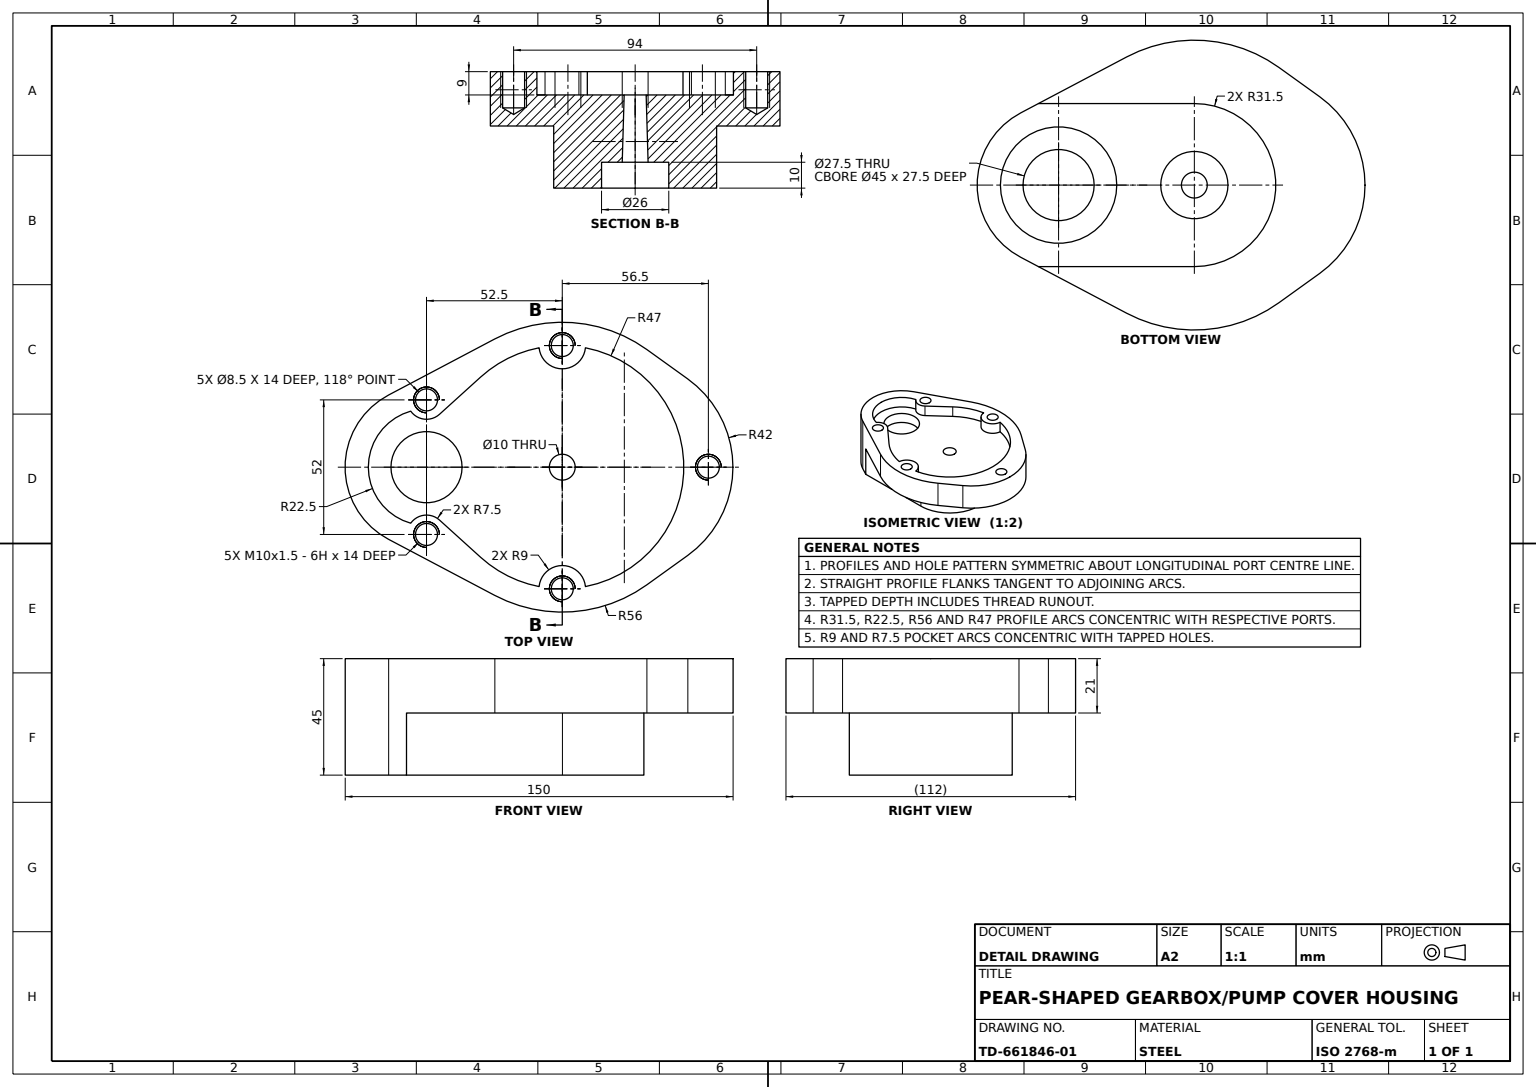
ISO-10303-21;
HEADER;
FILE_DESCRIPTION((''),'2;1');
FILE_NAME('','',(''),(''),'','','');
FILE_SCHEMA(('AUTOMOTIVE_DESIGN'));
ENDSEC;
DATA;
#1=APPLICATION_CONTEXT('');
#2=PRODUCT_CONTEXT('',#1,'mechanical');
#3=PRODUCT('','','',(#2));
#4=PRODUCT_DEFINITION_FORMATION('','',#3);
#5=PRODUCT_DEFINITION_CONTEXT('',#1,'design');
#6=PRODUCT_DEFINITION('','',#4,#5);
#7=PRODUCT_DEFINITION_SHAPE('','',#6);
#8=(LENGTH_UNIT()NAMED_UNIT(*)SI_UNIT(.MILLI.,.METRE.));
#9=(NAMED_UNIT(*)PLANE_ANGLE_UNIT()SI_UNIT($,.RADIAN.));
#10=(NAMED_UNIT(*)SI_UNIT($,.STERADIAN.)SOLID_ANGLE_UNIT());
#11=UNCERTAINTY_MEASURE_WITH_UNIT(LENGTH_MEASURE(1.E-05),#8,'distance_accuracy_value','');
#12=(GEOMETRIC_REPRESENTATION_CONTEXT(3)GLOBAL_UNCERTAINTY_ASSIGNED_CONTEXT((#11))GLOBAL_UNIT_ASSIGNED_CONTEXT((#8,#9,#10))REPRESENTATION_CONTEXT('',''));
#13=CARTESIAN_POINT('',(-26.,4.446342,0.));
#14=VERTEX_POINT('',#13);
#15=CARTESIAN_POINT('',(-26.,7.,4.25));
#16=VERTEX_POINT('',#15);
#17=DIRECTION('',(0.,0.515038075,0.857167301));
#18=VECTOR('',#17,1000.);
#19=LINE('',#15,#18);
#20=EDGE_CURVE('',#14,#16,#19,.T.);
#21=ORIENTED_EDGE('',*,*,#20,.T.);
#22=CARTESIAN_POINT('',(-26.,7.,-4.25));
#23=VERTEX_POINT('',#22);
#24=CARTESIAN_POINT('',(-26.,7.,0.));
#25=DIRECTION('',(0.,1.,0.));
#26=DIRECTION('',(0.,0.,1.));
#27=AXIS2_PLACEMENT_3D('',#24,#25,#26);
#28=CIRCLE('',#27,4.25);
#29=EDGE_CURVE('',#16,#23,#28,.T.);
#30=ORIENTED_EDGE('',*,*,#29,.T.);
#31=DIRECTION('',(0.,0.515038075,-0.857167301));
#32=VECTOR('',#31,1000.);
#33=LINE('',#22,#32);
#34=EDGE_CURVE('',#14,#23,#33,.T.);
#35=ORIENTED_EDGE('',*,*,#34,.F.);
#36=EDGE_LOOP('',(#21,#30,#35));
#37=FACE_OUTER_BOUND('',#36,.T.);
#38=CONICAL_SURFACE('',#27,4.25,1.029744259);
#39=ADVANCED_FACE('',(#37),#38,.F.);
#40=CARTESIAN_POINT('',(0.,21.,-104.75));
#41=VERTEX_POINT('',#40);
#42=CARTESIAN_POINT('',(0.,21.,-113.25));
#43=VERTEX_POINT('',#42);
#44=CARTESIAN_POINT('',(0.,21.,-109.));
#45=AXIS2_PLACEMENT_3D('',#44,#25,#26);
#46=CIRCLE('',#45,4.25);
#47=EDGE_CURVE('',#41,#43,#46,.T.);
#48=ORIENTED_EDGE('',*,*,#47,.T.);
#49=CARTESIAN_POINT('',(0.,7.,-113.25));
#50=VERTEX_POINT('',#49);
#51=VECTOR('',#25,1000.);
#52=LINE('',#42,#51);
#53=EDGE_CURVE('',#50,#43,#52,.T.);
#54=ORIENTED_EDGE('',*,*,#53,.F.);
#55=CARTESIAN_POINT('',(0.,7.,-104.75));
#56=VERTEX_POINT('',#55);
#57=CARTESIAN_POINT('',(0.,7.,-109.));
#58=AXIS2_PLACEMENT_3D('',#57,#25,#26);
#59=CIRCLE('',#58,4.25);
#60=EDGE_CURVE('',#56,#50,#59,.T.);
#61=ORIENTED_EDGE('',*,*,#60,.F.);
#62=LINE('',#40,#51);
#63=EDGE_CURVE('',#56,#41,#62,.T.);
#64=ORIENTED_EDGE('',*,*,#63,.T.);
#65=EDGE_LOOP('',(#48,#54,#61,#64));
#66=FACE_OUTER_BOUND('',#65,.T.);
#67=CYLINDRICAL_SURFACE('',#45,4.25);
#68=ADVANCED_FACE('',(#66),#67,.F.);
#69=CARTESIAN_POINT('',(0.,0.,-118.5));
#70=VERTEX_POINT('',#69);
#71=CARTESIAN_POINT('',(-34.11378,0.,-101.));
#72=VERTEX_POINT('',#71);
#73=CARTESIAN_POINT('',(0.,0.,-76.5));
#74=AXIS2_PLACEMENT_3D('',#73,#25,#26);
#75=CIRCLE('',#74,42.);
#76=EDGE_CURVE('',#70,#72,#75,.T.);
#77=ORIENTED_EDGE('',*,*,#76,.T.);
#78=CARTESIAN_POINT('',(-34.11378,21.,-101.));
#79=VERTEX_POINT('',#78);
#80=DIRECTION('',(0.,-1.,0.));
#81=VECTOR('',#80,1000.);
#82=LINE('',#78,#81);
#83=EDGE_CURVE('',#79,#72,#82,.T.);
#84=ORIENTED_EDGE('',*,*,#83,.F.);
#85=CARTESIAN_POINT('',(0.,21.,-118.5));
#86=VERTEX_POINT('',#85);
#87=CARTESIAN_POINT('',(0.,21.,-76.5));
#88=AXIS2_PLACEMENT_3D('',#87,#25,#26);
#89=CIRCLE('',#88,42.);
#90=EDGE_CURVE('',#86,#79,#89,.T.);
#91=ORIENTED_EDGE('',*,*,#90,.F.);
#92=LINE('',#85,#81);
#93=EDGE_CURVE('',#86,#70,#92,.T.);
#94=ORIENTED_EDGE('',*,*,#93,.T.);
#95=EDGE_LOOP('',(#77,#84,#91,#94));
#96=FACE_OUTER_BOUND('',#95,.T.);
#97=DIRECTION('',(0.,0.,-1.));
#98=AXIS2_PLACEMENT_3D('',#87,#80,#97);
#99=CYLINDRICAL_SURFACE('',#98,42.);
#100=ADVANCED_FACE('',(#96),#99,.T.);
#101=CARTESIAN_POINT('',(0.,12.,-47.5));
#102=VERTEX_POINT('',#101);
#103=CARTESIAN_POINT('',(0.,-14.,-47.5));
#104=VERTEX_POINT('',#103);
#105=CARTESIAN_POINT('',(0.,-24.,-47.5));
#106=LINE('',#105,#81);
#107=EDGE_CURVE('',#102,#104,#106,.T.);
#108=ORIENTED_EDGE('',*,*,#107,.T.);
#109=CARTESIAN_POINT('',(0.,-14.,-57.5));
#110=VERTEX_POINT('',#109);
#111=CARTESIAN_POINT('',(0.,-14.,-52.5));
#112=AXIS2_PLACEMENT_3D('',#111,#80,#97);
#113=CIRCLE('',#112,5.);
#114=EDGE_CURVE('',#104,#110,#113,.T.);
#115=ORIENTED_EDGE('',*,*,#114,.T.);
#116=CARTESIAN_POINT('',(0.,12.,-57.5));
#117=VERTEX_POINT('',#116);
#118=CARTESIAN_POINT('',(0.,-24.,-57.5));
#119=LINE('',#118,#81);
#120=EDGE_CURVE('',#117,#110,#119,.T.);
#121=ORIENTED_EDGE('',*,*,#120,.F.);
#122=CARTESIAN_POINT('',(0.,12.,-52.5));
#123=AXIS2_PLACEMENT_3D('',#122,#25,#26);
#124=CIRCLE('',#123,5.);
#125=EDGE_CURVE('',#117,#102,#124,.T.);
#126=ORIENTED_EDGE('',*,*,#125,.T.);
#127=EDGE_LOOP('',(#108,#115,#121,#126));
#128=FACE_OUTER_BOUND('',#127,.T.);
#129=CARTESIAN_POINT('',(0.,-24.,-52.5));
#130=AXIS2_PLACEMENT_3D('',#129,#80,#97);
#131=CYLINDRICAL_SURFACE('',#130,5.);
#132=ADVANCED_FACE('',(#128),#131,.F.);
#133=CARTESIAN_POINT('',(-47.,21.,-48.25));
#134=VERTEX_POINT('',#133);
#135=CARTESIAN_POINT('',(-47.,21.,-56.75));
#136=VERTEX_POINT('',#135);
#137=CARTESIAN_POINT('',(-47.,21.,-52.5));
#138=AXIS2_PLACEMENT_3D('',#137,#25,#26);
#139=CIRCLE('',#138,4.25);
#140=EDGE_CURVE('',#134,#136,#139,.T.);
#141=ORIENTED_EDGE('',*,*,#140,.T.);
#142=CARTESIAN_POINT('',(-47.,7.,-56.75));
#143=VERTEX_POINT('',#142);
#144=LINE('',#135,#51);
#145=EDGE_CURVE('',#143,#136,#144,.T.);
#146=ORIENTED_EDGE('',*,*,#145,.F.);
#147=CARTESIAN_POINT('',(-47.,7.,-48.25));
#148=VERTEX_POINT('',#147);
#149=CARTESIAN_POINT('',(-47.,7.,-52.5));
#150=AXIS2_PLACEMENT_3D('',#149,#25,#26);
#151=CIRCLE('',#150,4.25);
#152=EDGE_CURVE('',#148,#143,#151,.T.);
#153=ORIENTED_EDGE('',*,*,#152,.F.);
#154=LINE('',#133,#51);
#155=EDGE_CURVE('',#148,#134,#154,.T.);
#156=ORIENTED_EDGE('',*,*,#155,.T.);
#157=EDGE_LOOP('',(#141,#146,#153,#156));
#158=FACE_OUTER_BOUND('',#157,.T.);
#159=CYLINDRICAL_SURFACE('',#138,4.25);
#160=ADVANCED_FACE('',(#158),#159,.F.);
#161=CARTESIAN_POINT('',(-26.,21.,-4.25));
#162=VERTEX_POINT('',#161);
#163=LINE('',#161,#51);
#164=EDGE_CURVE('',#23,#162,#163,.T.);
#165=ORIENTED_EDGE('',*,*,#164,.T.);
#166=CARTESIAN_POINT('',(-26.,21.,4.25));
#167=VERTEX_POINT('',#166);
#168=CARTESIAN_POINT('',(-26.,21.,0.));
#169=AXIS2_PLACEMENT_3D('',#168,#25,#26);
#170=CIRCLE('',#169,4.25);
#171=EDGE_CURVE('',#162,#167,#170,.T.);
#172=ORIENTED_EDGE('',*,*,#171,.T.);
#173=LINE('',#166,#51);
#174=EDGE_CURVE('',#16,#167,#173,.T.);
#175=ORIENTED_EDGE('',*,*,#174,.F.);
#176=EDGE_CURVE('',#23,#16,#28,.T.);
#177=ORIENTED_EDGE('',*,*,#176,.F.);
#178=EDGE_LOOP('',(#165,#172,#175,#177));
#179=FACE_OUTER_BOUND('',#178,.T.);
#180=CYLINDRICAL_SURFACE('',#169,4.25);
#181=ADVANCED_FACE('',(#179),#180,.F.);
#182=CARTESIAN_POINT('',(-21.653846,12.,6.11236));
#183=VERTEX_POINT('',#182);
#184=CARTESIAN_POINT('',(0.,12.,22.5));
#185=VERTEX_POINT('',#184);
#186=CARTESIAN_POINT('',(0.,12.,0.));
#187=AXIS2_PLACEMENT_3D('',#186,#25,#26);
#188=CIRCLE('',#187,22.5);
#189=EDGE_CURVE('',#183,#185,#188,.T.);
#190=ORIENTED_EDGE('',*,*,#189,.F.);
#191=CARTESIAN_POINT('',(-21.653846,21.,6.11236));
#192=VERTEX_POINT('',#191);
#193=LINE('',#182,#51);
#194=EDGE_CURVE('',#183,#192,#193,.T.);
#195=ORIENTED_EDGE('',*,*,#194,.T.);
#196=CARTESIAN_POINT('',(0.,21.,22.5));
#197=VERTEX_POINT('',#196);
#198=CARTESIAN_POINT('',(0.,21.,0.));
#199=AXIS2_PLACEMENT_3D('',#198,#25,#26);
#200=CIRCLE('',#199,22.5);
#201=EDGE_CURVE('',#192,#197,#200,.T.);
#202=ORIENTED_EDGE('',*,*,#201,.T.);
#203=LINE('',#184,#51);
#204=EDGE_CURVE('',#185,#197,#203,.T.);
#205=ORIENTED_EDGE('',*,*,#204,.F.);
#206=EDGE_LOOP('',(#190,#195,#202,#205));
#207=FACE_OUTER_BOUND('',#206,.T.);
#208=CYLINDRICAL_SURFACE('',#187,22.5);
#209=ADVANCED_FACE('',(#207),#208,.F.);
#210=CARTESIAN_POINT('',(-49.528264,21.,-26.366667));
#211=VERTEX_POINT('',#210);
#212=CARTESIAN_POINT('',(-49.528264,0.,-26.366667));
#213=VERTEX_POINT('',#212);
#214=LINE('',#210,#81);
#215=EDGE_CURVE('',#211,#213,#214,.T.);
#216=ORIENTED_EDGE('',*,*,#215,.F.);
#217=CARTESIAN_POINT('',(-45.48504,21.,-85.166667));
#218=VERTEX_POINT('',#217);
#219=CARTESIAN_POINT('',(0.,21.,-52.5));
#220=AXIS2_PLACEMENT_3D('',#219,#25,#26);
#221=CIRCLE('',#220,56.);
#222=EDGE_CURVE('',#218,#211,#221,.T.);
#223=ORIENTED_EDGE('',*,*,#222,.F.);
#224=CARTESIAN_POINT('',(-45.48504,0.,-85.166667));
#225=VERTEX_POINT('',#224);
#226=LINE('',#217,#81);
#227=EDGE_CURVE('',#218,#225,#226,.T.);
#228=ORIENTED_EDGE('',*,*,#227,.T.);
#229=CARTESIAN_POINT('',(0.,0.,-52.5));
#230=AXIS2_PLACEMENT_3D('',#229,#25,#26);
#231=CIRCLE('',#230,56.);
#232=EDGE_CURVE('',#225,#213,#231,.T.);
#233=ORIENTED_EDGE('',*,*,#232,.T.);
#234=EDGE_LOOP('',(#216,#223,#228,#233));
#235=FACE_OUTER_BOUND('',#234,.T.);
#236=AXIS2_PLACEMENT_3D('',#219,#80,#97);
#237=CYLINDRICAL_SURFACE('',#236,56.);
#238=ADVANCED_FACE('',(#235),#237,.T.);
#239=ORIENTED_EDGE('',*,*,#204,.T.);
#240=CARTESIAN_POINT('',(21.653846,21.,6.11236));
#241=VERTEX_POINT('',#240);
#242=EDGE_CURVE('',#197,#241,#200,.T.);
#243=ORIENTED_EDGE('',*,*,#242,.T.);
#244=CARTESIAN_POINT('',(21.653846,12.,6.11236));
#245=VERTEX_POINT('',#244);
#246=LINE('',#244,#51);
#247=EDGE_CURVE('',#245,#241,#246,.T.);
#248=ORIENTED_EDGE('',*,*,#247,.F.);
#249=EDGE_CURVE('',#185,#245,#188,.T.);
#250=ORIENTED_EDGE('',*,*,#249,.F.);
#251=EDGE_LOOP('',(#239,#243,#248,#250));
#252=FACE_OUTER_BOUND('',#251,.T.);
#253=ADVANCED_FACE('',(#252),#208,.F.);
#254=CARTESIAN_POINT('',(-46.138298,12.,-43.541347));
#255=VERTEX_POINT('',#254);
#256=CARTESIAN_POINT('',(-46.138298,21.,-43.541347));
#257=VERTEX_POINT('',#256);
#258=LINE('',#254,#51);
#259=EDGE_CURVE('',#255,#257,#258,.T.);
#260=ORIENTED_EDGE('',*,*,#259,.T.);
#261=CARTESIAN_POINT('',(-34.856407,21.,-20.971744));
#262=VERTEX_POINT('',#261);
#263=CIRCLE('',#220,47.);
#264=EDGE_CURVE('',#257,#262,#263,.T.);
#265=ORIENTED_EDGE('',*,*,#264,.T.);
#266=CARTESIAN_POINT('',(-34.856407,12.,-20.971744));
#267=VERTEX_POINT('',#266);
#268=LINE('',#266,#51);
#269=EDGE_CURVE('',#267,#262,#268,.T.);
#270=ORIENTED_EDGE('',*,*,#269,.F.);
#271=CIRCLE('',#123,47.);
#272=EDGE_CURVE('',#255,#267,#271,.T.);
#273=ORIENTED_EDGE('',*,*,#272,.F.);
#274=EDGE_LOOP('',(#260,#265,#270,#273));
#275=FACE_OUTER_BOUND('',#274,.T.);
#276=CYLINDRICAL_SURFACE('',#123,47.);
#277=ADVANCED_FACE('',(#275),#276,.F.);
#278=CARTESIAN_POINT('',(26.,4.446342,0.));
#279=VERTEX_POINT('',#278);
#280=CARTESIAN_POINT('',(26.,7.,4.25));
#281=VERTEX_POINT('',#280);
#282=LINE('',#280,#18);
#283=EDGE_CURVE('',#279,#281,#282,.T.);
#284=ORIENTED_EDGE('',*,*,#283,.T.);
#285=CARTESIAN_POINT('',(26.,7.,-4.25));
#286=VERTEX_POINT('',#285);
#287=CARTESIAN_POINT('',(26.,7.,0.));
#288=AXIS2_PLACEMENT_3D('',#287,#25,#26);
#289=CIRCLE('',#288,4.25);
#290=EDGE_CURVE('',#281,#286,#289,.T.);
#291=ORIENTED_EDGE('',*,*,#290,.T.);
#292=LINE('',#285,#32);
#293=EDGE_CURVE('',#279,#286,#292,.T.);
#294=ORIENTED_EDGE('',*,*,#293,.F.);
#295=EDGE_LOOP('',(#284,#291,#294));
#296=FACE_OUTER_BOUND('',#295,.T.);
#297=CONICAL_SURFACE('',#288,4.25,1.029744259);
#298=ADVANCED_FACE('',(#296),#297,.F.);
#299=CARTESIAN_POINT('',(47.,7.,-56.75));
#300=VERTEX_POINT('',#299);
#301=CARTESIAN_POINT('',(47.,21.,-56.75));
#302=VERTEX_POINT('',#301);
#303=LINE('',#301,#51);
#304=EDGE_CURVE('',#300,#302,#303,.T.);
#305=ORIENTED_EDGE('',*,*,#304,.F.);
#306=CARTESIAN_POINT('',(47.,7.,-48.25));
#307=VERTEX_POINT('',#306);
#308=CARTESIAN_POINT('',(47.,7.,-52.5));
#309=AXIS2_PLACEMENT_3D('',#308,#25,#26);
#310=CIRCLE('',#309,4.25);
#311=EDGE_CURVE('',#307,#300,#310,.T.);
#312=ORIENTED_EDGE('',*,*,#311,.F.);
#313=CARTESIAN_POINT('',(47.,21.,-48.25));
#314=VERTEX_POINT('',#313);
#315=LINE('',#313,#51);
#316=EDGE_CURVE('',#307,#314,#315,.T.);
#317=ORIENTED_EDGE('',*,*,#316,.T.);
#318=CARTESIAN_POINT('',(47.,21.,-52.5));
#319=AXIS2_PLACEMENT_3D('',#318,#25,#26);
#320=CIRCLE('',#319,4.25);
#321=EDGE_CURVE('',#314,#302,#320,.T.);
#322=ORIENTED_EDGE('',*,*,#321,.T.);
#323=EDGE_LOOP('',(#305,#312,#317,#322));
#324=FACE_OUTER_BOUND('',#323,.T.);
#325=CYLINDRICAL_SURFACE('',#319,4.25);
#326=ADVANCED_FACE('',(#324),#325,.F.);
#327=CARTESIAN_POINT('',(0.,-24.,-65.5));
#328=VERTEX_POINT('',#327);
#329=CARTESIAN_POINT('',(0.,-24.,-39.5));
#330=VERTEX_POINT('',#329);
#331=CIRCLE('',#130,13.);
#332=EDGE_CURVE('',#328,#330,#331,.T.);
#333=ORIENTED_EDGE('',*,*,#332,.T.);
#334=CARTESIAN_POINT('',(0.,-14.,-39.5));
#335=VERTEX_POINT('',#334);
#336=LINE('',#329,#81);
#337=EDGE_CURVE('',#335,#330,#336,.T.);
#338=ORIENTED_EDGE('',*,*,#337,.F.);
#339=CARTESIAN_POINT('',(0.,-14.,-65.5));
#340=VERTEX_POINT('',#339);
#341=CIRCLE('',#112,13.);
#342=EDGE_CURVE('',#340,#335,#341,.T.);
#343=ORIENTED_EDGE('',*,*,#342,.F.);
#344=LINE('',#327,#81);
#345=EDGE_CURVE('',#340,#328,#344,.T.);
#346=ORIENTED_EDGE('',*,*,#345,.T.);
#347=EDGE_LOOP('',(#333,#338,#343,#346));
#348=FACE_OUTER_BOUND('',#347,.T.);
#349=CYLINDRICAL_SURFACE('',#130,13.);
#350=ADVANCED_FACE('',(#348),#349,.F.);
#351=CARTESIAN_POINT('',(0.,4.446342,-109.));
#352=VERTEX_POINT('',#351);
#353=LINE('',#55,#18);
#354=EDGE_CURVE('',#352,#56,#353,.T.);
#355=ORIENTED_EDGE('',*,*,#354,.F.);
#356=LINE('',#49,#32);
#357=EDGE_CURVE('',#352,#50,#356,.T.);
#358=ORIENTED_EDGE('',*,*,#357,.T.);
#359=EDGE_CURVE('',#50,#56,#59,.T.);
#360=ORIENTED_EDGE('',*,*,#359,.T.);
#361=EDGE_LOOP('',(#355,#358,#360));
#362=FACE_OUTER_BOUND('',#361,.T.);
#363=CONICAL_SURFACE('',#58,4.25,1.029744259);
#364=ADVANCED_FACE('',(#362),#363,.F.);
#365=CARTESIAN_POINT('',(-46.138298,12.,-61.458653));
#366=VERTEX_POINT('',#365);
#367=CARTESIAN_POINT('',(-47.,12.,-52.5));
#368=AXIS2_PLACEMENT_3D('',#367,#80,#26);
#369=CIRCLE('',#368,9.);
#370=EDGE_CURVE('',#366,#255,#369,.T.);
#371=ORIENTED_EDGE('',*,*,#370,.F.);
#372=CARTESIAN_POINT('',(-46.138298,21.,-61.458653));
#373=VERTEX_POINT('',#372);
#374=LINE('',#365,#51);
#375=EDGE_CURVE('',#366,#373,#374,.T.);
#376=ORIENTED_EDGE('',*,*,#375,.T.);
#377=AXIS2_PLACEMENT_3D('',#137,#80,#26);
#378=CIRCLE('',#377,9.);
#379=EDGE_CURVE('',#373,#257,#378,.T.);
#380=ORIENTED_EDGE('',*,*,#379,.T.);
#381=ORIENTED_EDGE('',*,*,#259,.F.);
#382=EDGE_LOOP('',(#371,#376,#380,#381));
#383=FACE_OUTER_BOUND('',#382,.T.);
#384=AXIS2_PLACEMENT_3D('',#367,#25,#26);
#385=CYLINDRICAL_SURFACE('',#384,9.);
#386=ADVANCED_FACE('',(#383),#385,.T.);
#387=ORIENTED_EDGE('',*,*,#120,.T.);
#388=EDGE_CURVE('',#110,#104,#113,.T.);
#389=ORIENTED_EDGE('',*,*,#388,.T.);
#390=ORIENTED_EDGE('',*,*,#107,.F.);
#391=EDGE_CURVE('',#102,#117,#124,.T.);
#392=ORIENTED_EDGE('',*,*,#391,.T.);
#393=EDGE_LOOP('',(#387,#389,#390,#392));
#394=FACE_OUTER_BOUND('',#393,.T.);
#395=ADVANCED_FACE('',(#394),#131,.F.);
#396=ORIENTED_EDGE('',*,*,#176,.T.);
#397=ORIENTED_EDGE('',*,*,#20,.F.);
#398=ORIENTED_EDGE('',*,*,#34,.T.);
#399=EDGE_LOOP('',(#396,#397,#398));
#400=FACE_OUTER_BOUND('',#399,.T.);
#401=ADVANCED_FACE('',(#400),#38,.F.);
#402=CARTESIAN_POINT('',(-47.,4.446342,-52.5));
#403=VERTEX_POINT('',#402);
#404=LINE('',#142,#32);
#405=EDGE_CURVE('',#403,#143,#404,.T.);
#406=ORIENTED_EDGE('',*,*,#405,.T.);
#407=EDGE_CURVE('',#143,#148,#151,.T.);
#408=ORIENTED_EDGE('',*,*,#407,.T.);
#409=LINE('',#147,#18);
#410=EDGE_CURVE('',#403,#148,#409,.T.);
#411=ORIENTED_EDGE('',*,*,#410,.F.);
#412=EDGE_LOOP('',(#406,#408,#411));
#413=FACE_OUTER_BOUND('',#412,.T.);
#414=CONICAL_SURFACE('',#150,4.25,1.029744259);
#415=ADVANCED_FACE('',(#413),#414,.F.);
#416=ORIENTED_EDGE('',*,*,#227,.F.);
#417=DIRECTION('',(-0.583333333,0.,0.812232862));
#418=VECTOR('',#417,1000.);
#419=LINE('',#217,#418);
#420=EDGE_CURVE('',#79,#218,#419,.T.);
#421=ORIENTED_EDGE('',*,*,#420,.F.);
#422=ORIENTED_EDGE('',*,*,#83,.T.);
#423=LINE('',#224,#418);
#424=EDGE_CURVE('',#72,#225,#423,.T.);
#425=ORIENTED_EDGE('',*,*,#424,.T.);
#426=EDGE_LOOP('',(#416,#421,#422,#425));
#427=FACE_OUTER_BOUND('',#426,.T.);
#428=DIRECTION('',(0.812232862,0.,0.583333333));
#429=DIRECTION('',(0.583333333,0.,-0.812232862));
#430=AXIS2_PLACEMENT_3D('',#217,#428,#429);
#431=PLANE('',#430);
#432=ADVANCED_FACE('',(#427),#431,.F.);
#433=ORIENTED_EDGE('',*,*,#332,.F.);
#434=EDGE_CURVE('',#330,#328,#331,.T.);
#435=ORIENTED_EDGE('',*,*,#434,.F.);
#436=EDGE_LOOP('',(#433,#435));
#437=FACE_BOUND('',#436,.T.);
#438=CARTESIAN_POINT('',(0.,-24.,-22.5));
#439=VERTEX_POINT('',#438);
#440=CARTESIAN_POINT('',(0.,-24.,22.5));
#441=VERTEX_POINT('',#440);
#442=CARTESIAN_POINT('',(0.,-24.,0.));
#443=AXIS2_PLACEMENT_3D('',#442,#80,#97);
#444=CIRCLE('',#443,22.5);
#445=EDGE_CURVE('',#439,#441,#444,.T.);
#446=ORIENTED_EDGE('',*,*,#445,.F.);
#447=EDGE_CURVE('',#441,#439,#444,.T.);
#448=ORIENTED_EDGE('',*,*,#447,.F.);
#449=EDGE_LOOP('',(#446,#448));
#450=FACE_BOUND('',#449,.T.);
#451=CARTESIAN_POINT('',(-27.859648,-24.,14.7));
#452=VERTEX_POINT('',#451);
#453=CARTESIAN_POINT('',(-31.5,-24.,7.800754));
#454=VERTEX_POINT('',#453);
#455=DIRECTION('',(-0.466666667,0.,-0.884433277));
#456=VECTOR('',#455,1000.);
#457=LINE('',#453,#456);
#458=EDGE_CURVE('',#452,#454,#457,.T.);
#459=ORIENTED_EDGE('',*,*,#458,.T.);
#460=CARTESIAN_POINT('',(-31.5,-24.,-52.5));
#461=VERTEX_POINT('',#460);
#462=CARTESIAN_POINT('',(-31.5,-24.,0.));
#463=VECTOR('',#97,1000.);
#464=LINE('',#462,#463);
#465=EDGE_CURVE('',#454,#461,#464,.T.);
#466=ORIENTED_EDGE('',*,*,#465,.T.);
#467=CARTESIAN_POINT('',(31.5,-24.,-52.5));
#468=VERTEX_POINT('',#467);
#469=CIRCLE('',#130,31.5);
#470=EDGE_CURVE('',#461,#468,#469,.T.);
#471=ORIENTED_EDGE('',*,*,#470,.T.);
#472=CARTESIAN_POINT('',(31.5,-24.,7.800754));
#473=VERTEX_POINT('',#472);
#474=CARTESIAN_POINT('',(31.5,-24.,0.));
#475=VECTOR('',#26,1000.);
#476=LINE('',#474,#475);
#477=EDGE_CURVE('',#468,#473,#476,.T.);
#478=ORIENTED_EDGE('',*,*,#477,.T.);
#479=CARTESIAN_POINT('',(27.859648,-24.,14.7));
#480=VERTEX_POINT('',#479);
#481=DIRECTION('',(-0.466666667,0.,0.884433277));
#482=VECTOR('',#481,1000.);
#483=LINE('',#479,#482);
#484=EDGE_CURVE('',#473,#480,#483,.T.);
#485=ORIENTED_EDGE('',*,*,#484,.T.);
#486=CIRCLE('',#443,31.5);
#487=EDGE_CURVE('',#480,#452,#486,.T.);
#488=ORIENTED_EDGE('',*,*,#487,.T.);
#489=EDGE_LOOP('',(#459,#466,#471,#478,#485,#488));
#490=FACE_OUTER_BOUND('',#489,.T.);
#491=PLANE('',#443);
#492=ADVANCED_FACE('',(#437,#450,#490),#491,.T.);
#493=CARTESIAN_POINT('',(47.,4.446342,-52.5));
#494=VERTEX_POINT('',#493);
#495=LINE('',#306,#18);
#496=EDGE_CURVE('',#494,#307,#495,.T.);
#497=ORIENTED_EDGE('',*,*,#496,.F.);
#498=LINE('',#299,#32);
#499=EDGE_CURVE('',#494,#300,#498,.T.);
#500=ORIENTED_EDGE('',*,*,#499,.T.);
#501=EDGE_CURVE('',#300,#307,#310,.T.);
#502=ORIENTED_EDGE('',*,*,#501,.T.);
#503=EDGE_LOOP('',(#497,#500,#502));
#504=FACE_OUTER_BOUND('',#503,.T.);
#505=CONICAL_SURFACE('',#309,4.25,1.029744259);
#506=ADVANCED_FACE('',(#504),#505,.F.);
#507=CARTESIAN_POINT('',(0.,3.5,22.5));
#508=VERTEX_POINT('',#507);
#509=LINE('',#440,#81);
#510=EDGE_CURVE('',#508,#441,#509,.T.);
#511=ORIENTED_EDGE('',*,*,#510,.F.);
#512=CARTESIAN_POINT('',(0.,3.5,-22.5));
#513=VERTEX_POINT('',#512);
#514=CARTESIAN_POINT('',(0.,3.5,0.));
#515=AXIS2_PLACEMENT_3D('',#514,#80,#97);
#516=CIRCLE('',#515,22.5);
#517=EDGE_CURVE('',#513,#508,#516,.T.);
#518=ORIENTED_EDGE('',*,*,#517,.F.);
#519=LINE('',#438,#81);
#520=EDGE_CURVE('',#513,#439,#519,.T.);
#521=ORIENTED_EDGE('',*,*,#520,.T.);
#522=ORIENTED_EDGE('',*,*,#445,.T.);
#523=EDGE_LOOP('',(#511,#518,#521,#522));
#524=FACE_OUTER_BOUND('',#523,.T.);
#525=CYLINDRICAL_SURFACE('',#443,22.5);
#526=ADVANCED_FACE('',(#524),#525,.F.);
#527=EDGE_CURVE('',#286,#281,#289,.T.);
#528=ORIENTED_EDGE('',*,*,#527,.T.);
#529=ORIENTED_EDGE('',*,*,#283,.F.);
#530=ORIENTED_EDGE('',*,*,#293,.T.);
#531=EDGE_LOOP('',(#528,#529,#530));
#532=FACE_OUTER_BOUND('',#531,.T.);
#533=ADVANCED_FACE('',(#532),#297,.F.);
#534=CARTESIAN_POINT('',(45.48504,0.,-85.166667));
#535=VERTEX_POINT('',#534);
#536=CARTESIAN_POINT('',(34.11378,0.,-101.));
#537=VERTEX_POINT('',#536);
#538=DIRECTION('',(-0.583333333,0.,-0.812232862));
#539=VECTOR('',#538,1000.);
#540=LINE('',#534,#539);
#541=EDGE_CURVE('',#535,#537,#540,.T.);
#542=ORIENTED_EDGE('',*,*,#541,.F.);
#543=CARTESIAN_POINT('',(49.528264,0.,-26.366667));
#544=VERTEX_POINT('',#543);
#545=EDGE_CURVE('',#544,#535,#231,.T.);
#546=ORIENTED_EDGE('',*,*,#545,.F.);
#547=CARTESIAN_POINT('',(31.5,0.,7.800754));
#548=VERTEX_POINT('',#547);
#549=CARTESIAN_POINT('',(27.859648,0.,14.7));
#550=DIRECTION('',(0.466666667,0.,-0.884433277));
#551=VECTOR('',#550,1000.);
#552=LINE('',#549,#551);
#553=EDGE_CURVE('',#548,#544,#552,.T.);
#554=ORIENTED_EDGE('',*,*,#553,.F.);
#555=CARTESIAN_POINT('',(31.5,0.,-52.5));
#556=VERTEX_POINT('',#555);
#557=CARTESIAN_POINT('',(31.5,0.,0.));
#558=LINE('',#557,#475);
#559=EDGE_CURVE('',#556,#548,#558,.T.);
#560=ORIENTED_EDGE('',*,*,#559,.F.);
#561=CARTESIAN_POINT('',(-31.5,0.,-52.5));
#562=VERTEX_POINT('',#561);
#563=AXIS2_PLACEMENT_3D('',#229,#80,#97);
#564=CIRCLE('',#563,31.5);
#565=EDGE_CURVE('',#562,#556,#564,.T.);
#566=ORIENTED_EDGE('',*,*,#565,.F.);
#567=CARTESIAN_POINT('',(-31.5,0.,7.800754));
#568=VERTEX_POINT('',#567);
#569=CARTESIAN_POINT('',(-31.5,0.,0.));
#570=LINE('',#569,#463);
#571=EDGE_CURVE('',#568,#562,#570,.T.);
#572=ORIENTED_EDGE('',*,*,#571,.F.);
#573=DIRECTION('',(0.466666667,0.,0.884433277));
#574=VECTOR('',#573,1000.);
#575=LINE('',#212,#574);
#576=EDGE_CURVE('',#213,#568,#575,.T.);
#577=ORIENTED_EDGE('',*,*,#576,.F.);
#578=ORIENTED_EDGE('',*,*,#232,.F.);
#579=ORIENTED_EDGE('',*,*,#424,.F.);
#580=ORIENTED_EDGE('',*,*,#76,.F.);
#581=EDGE_CURVE('',#537,#70,#75,.T.);
#582=ORIENTED_EDGE('',*,*,#581,.F.);
#583=EDGE_LOOP('',(#542,#546,#554,#560,#566,#572,#577,#578,#579,#580,#582));
#584=FACE_OUTER_BOUND('',#583,.T.);
#585=CARTESIAN_POINT('',(0.,0.,0.));
#586=AXIS2_PLACEMENT_3D('',#585,#25,#26);
#587=PLANE('',#586);
#588=ADVANCED_FACE('',(#584),#587,.F.);
#589=CARTESIAN_POINT('',(0.,3.5,13.75));
#590=VERTEX_POINT('',#589);
#591=CARTESIAN_POINT('',(0.,3.5,-13.75));
#592=VERTEX_POINT('',#591);
#593=CIRCLE('',#515,13.75);
#594=EDGE_CURVE('',#590,#592,#593,.T.);
#595=ORIENTED_EDGE('',*,*,#594,.T.);
#596=CARTESIAN_POINT('',(0.,12.,-13.75));
#597=VERTEX_POINT('',#596);
#598=CARTESIAN_POINT('',(0.,-24.,-13.75));
#599=LINE('',#598,#81);
#600=EDGE_CURVE('',#597,#592,#599,.T.);
#601=ORIENTED_EDGE('',*,*,#600,.F.);
#602=CARTESIAN_POINT('',(0.,12.,13.75));
#603=VERTEX_POINT('',#602);
#604=CIRCLE('',#187,13.75);
#605=EDGE_CURVE('',#597,#603,#604,.T.);
#606=ORIENTED_EDGE('',*,*,#605,.T.);
#607=CARTESIAN_POINT('',(0.,-24.,13.75));
#608=LINE('',#607,#81);
#609=EDGE_CURVE('',#603,#590,#608,.T.);
#610=ORIENTED_EDGE('',*,*,#609,.T.);
#611=EDGE_LOOP('',(#595,#601,#606,#610));
#612=FACE_OUTER_BOUND('',#611,.T.);
#613=CYLINDRICAL_SURFACE('',#443,13.75);
#614=ADVANCED_FACE('',(#612),#613,.F.);
#615=ORIENTED_EDGE('',*,*,#63,.F.);
#616=ORIENTED_EDGE('',*,*,#359,.F.);
#617=ORIENTED_EDGE('',*,*,#53,.T.);
#618=EDGE_CURVE('',#43,#41,#46,.T.);
#619=ORIENTED_EDGE('',*,*,#618,.T.);
#620=EDGE_LOOP('',(#615,#616,#617,#619));
#621=FACE_OUTER_BOUND('',#620,.T.);
#622=ADVANCED_FACE('',(#621),#67,.F.);
#623=CARTESIAN_POINT('',(46.138298,12.,-43.541347));
#624=VERTEX_POINT('',#623);
#625=CARTESIAN_POINT('',(46.138298,21.,-43.541347));
#626=VERTEX_POINT('',#625);
#627=LINE('',#623,#51);
#628=EDGE_CURVE('',#624,#626,#627,.T.);
#629=ORIENTED_EDGE('',*,*,#628,.F.);
#630=CARTESIAN_POINT('',(34.856407,12.,-20.971744));
#631=VERTEX_POINT('',#630);
#632=EDGE_CURVE('',#631,#624,#271,.T.);
#633=ORIENTED_EDGE('',*,*,#632,.F.);
#634=CARTESIAN_POINT('',(34.856407,21.,-20.971744));
#635=VERTEX_POINT('',#634);
#636=LINE('',#630,#51);
#637=EDGE_CURVE('',#631,#635,#636,.T.);
#638=ORIENTED_EDGE('',*,*,#637,.T.);
#639=EDGE_CURVE('',#635,#626,#263,.T.);
#640=ORIENTED_EDGE('',*,*,#639,.T.);
#641=EDGE_LOOP('',(#629,#633,#638,#640));
#642=FACE_OUTER_BOUND('',#641,.T.);
#643=ADVANCED_FACE('',(#642),#276,.F.);
#644=ORIENTED_EDGE('',*,*,#174,.T.);
#645=EDGE_CURVE('',#167,#162,#170,.T.);
#646=ORIENTED_EDGE('',*,*,#645,.T.);
#647=ORIENTED_EDGE('',*,*,#164,.F.);
#648=ORIENTED_EDGE('',*,*,#29,.F.);
#649=EDGE_LOOP('',(#644,#646,#647,#648));
#650=FACE_OUTER_BOUND('',#649,.T.);
#651=ADVANCED_FACE('',(#650),#180,.F.);
#652=ORIENTED_EDGE('',*,*,#311,.T.);
#653=ORIENTED_EDGE('',*,*,#499,.F.);
#654=ORIENTED_EDGE('',*,*,#496,.T.);
#655=EDGE_LOOP('',(#652,#653,#654));
#656=FACE_OUTER_BOUND('',#655,.T.);
#657=ADVANCED_FACE('',(#656),#505,.F.);
#658=CARTESIAN_POINT('',(-20.437807,21.,-5.031105));
#659=VERTEX_POINT('',#658);
#660=CARTESIAN_POINT('',(-21.596473,21.,-6.31208));
#661=DIRECTION('',(0.670813951,0.,0.741625676));
#662=VECTOR('',#661,1000.);
#663=LINE('',#660,#662);
#664=EDGE_CURVE('',#262,#659,#663,.T.);
#665=ORIENTED_EDGE('',*,*,#664,.T.);
#666=CARTESIAN_POINT('',(-20.437807,12.,-5.031105));
#667=VERTEX_POINT('',#666);
#668=LINE('',#666,#51);
#669=EDGE_CURVE('',#667,#659,#668,.T.);
#670=ORIENTED_EDGE('',*,*,#669,.F.);
#671=LINE('',#266,#662);
#672=EDGE_CURVE('',#267,#667,#671,.T.);
#673=ORIENTED_EDGE('',*,*,#672,.F.);
#674=ORIENTED_EDGE('',*,*,#269,.T.);
#675=EDGE_LOOP('',(#665,#670,#673,#674));
#676=FACE_OUTER_BOUND('',#675,.T.);
#677=CARTESIAN_POINT('',(-21.596473,12.,-6.31208));
#678=DIRECTION('',(-0.741625676,0.,0.670813951));
#679=AXIS2_PLACEMENT_3D('',#677,#678,#661);
#680=PLANE('',#679);
#681=ADVANCED_FACE('',(#676),#680,.F.);
#682=EDGE_CURVE('',#302,#314,#320,.T.);
#683=ORIENTED_EDGE('',*,*,#682,.T.);
#684=ORIENTED_EDGE('',*,*,#316,.F.);
#685=ORIENTED_EDGE('',*,*,#501,.F.);
#686=ORIENTED_EDGE('',*,*,#304,.T.);
#687=EDGE_LOOP('',(#683,#684,#685,#686));
#688=FACE_OUTER_BOUND('',#687,.T.);
#689=ADVANCED_FACE('',(#688),#325,.F.);
#690=ORIENTED_EDGE('',*,*,#559,.T.);
#691=LINE('',#472,#51);
#692=EDGE_CURVE('',#473,#548,#691,.T.);
#693=ORIENTED_EDGE('',*,*,#692,.F.);
#694=ORIENTED_EDGE('',*,*,#477,.F.);
#695=LINE('',#467,#51);
#696=EDGE_CURVE('',#468,#556,#695,.T.);
#697=ORIENTED_EDGE('',*,*,#696,.T.);
#698=EDGE_LOOP('',(#690,#693,#694,#697));
#699=FACE_OUTER_BOUND('',#698,.T.);
#700=DIRECTION('',(-1.,0.,0.));
#701=AXIS2_PLACEMENT_3D('',#474,#700,#26);
#702=PLANE('',#701);
#703=ADVANCED_FACE('',(#699),#702,.F.);
#704=ORIENTED_EDGE('',*,*,#527,.F.);
#705=CARTESIAN_POINT('',(26.,21.,-4.25));
#706=VERTEX_POINT('',#705);
#707=LINE('',#705,#51);
#708=EDGE_CURVE('',#286,#706,#707,.T.);
#709=ORIENTED_EDGE('',*,*,#708,.T.);
#710=CARTESIAN_POINT('',(26.,21.,4.25));
#711=VERTEX_POINT('',#710);
#712=CARTESIAN_POINT('',(26.,21.,0.));
#713=AXIS2_PLACEMENT_3D('',#712,#25,#26);
#714=CIRCLE('',#713,4.25);
#715=EDGE_CURVE('',#706,#711,#714,.T.);
#716=ORIENTED_EDGE('',*,*,#715,.T.);
#717=LINE('',#710,#51);
#718=EDGE_CURVE('',#281,#711,#717,.T.);
#719=ORIENTED_EDGE('',*,*,#718,.F.);
#720=EDGE_LOOP('',(#704,#709,#716,#719));
#721=FACE_OUTER_BOUND('',#720,.T.);
#722=CYLINDRICAL_SURFACE('',#713,4.25);
#723=ADVANCED_FACE('',(#721),#722,.F.);
#724=ORIENTED_EDGE('',*,*,#541,.T.);
#725=CARTESIAN_POINT('',(34.11378,21.,-101.));
#726=VERTEX_POINT('',#725);
#727=LINE('',#725,#81);
#728=EDGE_CURVE('',#726,#537,#727,.T.);
#729=ORIENTED_EDGE('',*,*,#728,.F.);
#730=CARTESIAN_POINT('',(45.48504,21.,-85.166667));
#731=VERTEX_POINT('',#730);
#732=LINE('',#730,#539);
#733=EDGE_CURVE('',#731,#726,#732,.T.);
#734=ORIENTED_EDGE('',*,*,#733,.F.);
#735=LINE('',#730,#81);
#736=EDGE_CURVE('',#731,#535,#735,.T.);
#737=ORIENTED_EDGE('',*,*,#736,.T.);
#738=EDGE_LOOP('',(#724,#729,#734,#737));
#739=FACE_OUTER_BOUND('',#738,.T.);
#740=DIRECTION('',(-0.812232862,0.,0.583333333));
#741=DIRECTION('',(0.583333333,0.,0.812232862));
#742=AXIS2_PLACEMENT_3D('',#730,#740,#741);
#743=PLANE('',#742);
#744=ADVANCED_FACE('',(#739),#743,.F.);
#745=CARTESIAN_POINT('',(20.437807,12.,-5.031105));
#746=VERTEX_POINT('',#745);
#747=CARTESIAN_POINT('',(20.437807,21.,-5.031105));
#748=VERTEX_POINT('',#747);
#749=LINE('',#745,#51);
#750=EDGE_CURVE('',#746,#748,#749,.T.);
#751=ORIENTED_EDGE('',*,*,#750,.F.);
#752=CARTESIAN_POINT('',(26.,12.,0.));
#753=AXIS2_PLACEMENT_3D('',#752,#80,#97);
#754=CIRCLE('',#753,7.5);
#755=EDGE_CURVE('',#245,#746,#754,.T.);
#756=ORIENTED_EDGE('',*,*,#755,.F.);
#757=ORIENTED_EDGE('',*,*,#247,.T.);
#758=AXIS2_PLACEMENT_3D('',#712,#80,#97);
#759=CIRCLE('',#758,7.5);
#760=EDGE_CURVE('',#241,#748,#759,.T.);
#761=ORIENTED_EDGE('',*,*,#760,.T.);
#762=EDGE_LOOP('',(#751,#756,#757,#761));
#763=FACE_OUTER_BOUND('',#762,.T.);
#764=AXIS2_PLACEMENT_3D('',#752,#25,#26);
#765=CYLINDRICAL_SURFACE('',#764,7.5);
#766=ADVANCED_FACE('',(#763),#765,.T.);
#767=LINE('',#460,#51);
#768=EDGE_CURVE('',#461,#562,#767,.T.);
#769=ORIENTED_EDGE('',*,*,#768,.T.);
#770=ORIENTED_EDGE('',*,*,#565,.T.);
#771=ORIENTED_EDGE('',*,*,#696,.F.);
#772=ORIENTED_EDGE('',*,*,#470,.F.);
#773=EDGE_LOOP('',(#769,#770,#771,#772));
#774=FACE_OUTER_BOUND('',#773,.T.);
#775=AXIS2_PLACEMENT_3D('',#129,#25,#26);
#776=CYLINDRICAL_SURFACE('',#775,31.5);
#777=ADVANCED_FACE('',(#774),#776,.T.);
#778=CARTESIAN_POINT('',(-26.,12.,0.));
#779=AXIS2_PLACEMENT_3D('',#778,#80,#26);
#780=CIRCLE('',#779,7.5);
#781=EDGE_CURVE('',#667,#183,#780,.T.);
#782=ORIENTED_EDGE('',*,*,#781,.T.);
#783=ORIENTED_EDGE('',*,*,#189,.T.);
#784=ORIENTED_EDGE('',*,*,#249,.T.);
#785=ORIENTED_EDGE('',*,*,#755,.T.);
#786=DIRECTION('',(0.670813951,0.,-0.741625676));
#787=VECTOR('',#786,1000.);
#788=LINE('',#630,#787);
#789=EDGE_CURVE('',#746,#631,#788,.T.);
#790=ORIENTED_EDGE('',*,*,#789,.T.);
#791=ORIENTED_EDGE('',*,*,#632,.T.);
#792=CARTESIAN_POINT('',(46.138298,12.,-61.458653));
#793=VERTEX_POINT('',#792);
#794=CARTESIAN_POINT('',(47.,12.,-52.5));
#795=AXIS2_PLACEMENT_3D('',#794,#80,#97);
#796=CIRCLE('',#795,9.);
#797=EDGE_CURVE('',#624,#793,#796,.T.);
#798=ORIENTED_EDGE('',*,*,#797,.T.);
#799=EDGE_CURVE('',#793,#366,#271,.T.);
#800=ORIENTED_EDGE('',*,*,#799,.T.);
#801=ORIENTED_EDGE('',*,*,#370,.T.);
#802=ORIENTED_EDGE('',*,*,#272,.T.);
#803=ORIENTED_EDGE('',*,*,#672,.T.);
#804=EDGE_LOOP('',(#782,#783,#784,#785,#790,#791,#798,#800,#801,#802,#803));
#805=FACE_OUTER_BOUND('',#804,.T.);
#806=ORIENTED_EDGE('',*,*,#605,.F.);
#807=EDGE_CURVE('',#603,#597,#604,.T.);
#808=ORIENTED_EDGE('',*,*,#807,.F.);
#809=EDGE_LOOP('',(#806,#808));
#810=FACE_BOUND('',#809,.T.);
#811=ORIENTED_EDGE('',*,*,#391,.F.);
#812=ORIENTED_EDGE('',*,*,#125,.F.);
#813=EDGE_LOOP('',(#811,#812));
#814=FACE_BOUND('',#813,.T.);
#815=PLANE('',#123);
#816=ADVANCED_FACE('',(#805,#810,#814),#815,.T.);
#817=ORIENTED_EDGE('',*,*,#637,.F.);
#818=ORIENTED_EDGE('',*,*,#789,.F.);
#819=ORIENTED_EDGE('',*,*,#750,.T.);
#820=LINE('',#634,#787);
#821=EDGE_CURVE('',#748,#635,#820,.T.);
#822=ORIENTED_EDGE('',*,*,#821,.T.);
#823=EDGE_LOOP('',(#817,#818,#819,#822));
#824=FACE_OUTER_BOUND('',#823,.T.);
#825=DIRECTION('',(0.741625676,0.,0.670813951));
#826=AXIS2_PLACEMENT_3D('',#630,#825,#786);
#827=PLANE('',#826);
#828=ADVANCED_FACE('',(#824),#827,.F.);
#829=ORIENTED_EDGE('',*,*,#357,.F.);
#830=ORIENTED_EDGE('',*,*,#354,.T.);
#831=ORIENTED_EDGE('',*,*,#60,.T.);
#832=EDGE_LOOP('',(#829,#830,#831));
#833=FACE_OUTER_BOUND('',#832,.T.);
#834=ADVANCED_FACE('',(#833),#363,.F.);
#835=ORIENTED_EDGE('',*,*,#345,.F.);
#836=EDGE_CURVE('',#335,#340,#341,.T.);
#837=ORIENTED_EDGE('',*,*,#836,.F.);
#838=ORIENTED_EDGE('',*,*,#337,.T.);
#839=ORIENTED_EDGE('',*,*,#434,.T.);
#840=EDGE_LOOP('',(#835,#837,#838,#839));
#841=FACE_OUTER_BOUND('',#840,.T.);
#842=ADVANCED_FACE('',(#841),#349,.F.);
#843=CARTESIAN_POINT('',(-27.859648,21.,14.7));
#844=VERTEX_POINT('',#843);
#845=LINE('',#210,#574);
#846=EDGE_CURVE('',#211,#844,#845,.T.);
#847=ORIENTED_EDGE('',*,*,#846,.F.);
#848=ORIENTED_EDGE('',*,*,#215,.T.);
#849=ORIENTED_EDGE('',*,*,#576,.T.);
#850=LINE('',#453,#51);
#851=EDGE_CURVE('',#454,#568,#850,.T.);
#852=ORIENTED_EDGE('',*,*,#851,.F.);
#853=ORIENTED_EDGE('',*,*,#458,.F.);
#854=LINE('',#843,#81);
#855=EDGE_CURVE('',#844,#452,#854,.T.);
#856=ORIENTED_EDGE('',*,*,#855,.F.);
#857=EDGE_LOOP('',(#847,#848,#849,#852,#853,#856));
#858=FACE_OUTER_BOUND('',#857,.T.);
#859=DIRECTION('',(0.884433277,0.,-0.466666667));
#860=AXIS2_PLACEMENT_3D('',#210,#859,#455);
#861=PLANE('',#860);
#862=ADVANCED_FACE('',(#858),#861,.F.);
#863=ORIENTED_EDGE('',*,*,#375,.F.);
#864=ORIENTED_EDGE('',*,*,#799,.F.);
#865=CARTESIAN_POINT('',(46.138298,21.,-61.458653));
#866=VERTEX_POINT('',#865);
#867=LINE('',#792,#51);
#868=EDGE_CURVE('',#793,#866,#867,.T.);
#869=ORIENTED_EDGE('',*,*,#868,.T.);
#870=EDGE_CURVE('',#866,#373,#263,.T.);
#871=ORIENTED_EDGE('',*,*,#870,.T.);
#872=EDGE_LOOP('',(#863,#864,#869,#871));
#873=FACE_OUTER_BOUND('',#872,.T.);
#874=ADVANCED_FACE('',(#873),#276,.F.);
#875=ORIENTED_EDGE('',*,*,#571,.T.);
#876=ORIENTED_EDGE('',*,*,#768,.F.);
#877=ORIENTED_EDGE('',*,*,#465,.F.);
#878=ORIENTED_EDGE('',*,*,#851,.T.);
#879=EDGE_LOOP('',(#875,#876,#877,#878));
#880=FACE_OUTER_BOUND('',#879,.T.);
#881=DIRECTION('',(1.,0.,0.));
#882=AXIS2_PLACEMENT_3D('',#462,#881,#97);
#883=PLANE('',#882);
#884=ADVANCED_FACE('',(#880),#883,.F.);
#885=EDGE_CURVE('',#592,#590,#593,.T.);
#886=ORIENTED_EDGE('',*,*,#885,.F.);
#887=ORIENTED_EDGE('',*,*,#594,.F.);
#888=EDGE_LOOP('',(#886,#887));
#889=FACE_BOUND('',#888,.T.);
#890=EDGE_CURVE('',#508,#513,#516,.T.);
#891=ORIENTED_EDGE('',*,*,#890,.T.);
#892=ORIENTED_EDGE('',*,*,#517,.T.);
#893=EDGE_LOOP('',(#891,#892));
#894=FACE_OUTER_BOUND('',#893,.T.);
#895=CARTESIAN_POINT('',(13.75,3.5,0.));
#896=AXIS2_PLACEMENT_3D('',#895,#25,#26);
#897=PLANE('',#896);
#898=ADVANCED_FACE('',(#889,#894),#897,.F.);
#899=ORIENTED_EDGE('',*,*,#484,.F.);
#900=ORIENTED_EDGE('',*,*,#692,.T.);
#901=ORIENTED_EDGE('',*,*,#553,.T.);
#902=CARTESIAN_POINT('',(49.528264,21.,-26.366667));
#903=VERTEX_POINT('',#902);
#904=LINE('',#902,#81);
#905=EDGE_CURVE('',#903,#544,#904,.T.);
#906=ORIENTED_EDGE('',*,*,#905,.F.);
#907=CARTESIAN_POINT('',(27.859648,21.,14.7));
#908=VERTEX_POINT('',#907);
#909=LINE('',#907,#551);
#910=EDGE_CURVE('',#908,#903,#909,.T.);
#911=ORIENTED_EDGE('',*,*,#910,.F.);
#912=LINE('',#907,#81);
#913=EDGE_CURVE('',#908,#480,#912,.T.);
#914=ORIENTED_EDGE('',*,*,#913,.T.);
#915=EDGE_LOOP('',(#899,#900,#901,#906,#911,#914));
#916=FACE_OUTER_BOUND('',#915,.T.);
#917=DIRECTION('',(-0.884433277,0.,-0.466666667));
#918=AXIS2_PLACEMENT_3D('',#907,#917,#481);
#919=PLANE('',#918);
#920=ADVANCED_FACE('',(#916),#919,.F.);
#921=ORIENTED_EDGE('',*,*,#600,.T.);
#922=ORIENTED_EDGE('',*,*,#885,.T.);
#923=ORIENTED_EDGE('',*,*,#609,.F.);
#924=ORIENTED_EDGE('',*,*,#807,.T.);
#925=EDGE_LOOP('',(#921,#922,#923,#924));
#926=FACE_OUTER_BOUND('',#925,.T.);
#927=ADVANCED_FACE('',(#926),#613,.F.);
#928=ORIENTED_EDGE('',*,*,#152,.T.);
#929=ORIENTED_EDGE('',*,*,#405,.F.);
#930=ORIENTED_EDGE('',*,*,#410,.T.);
#931=EDGE_LOOP('',(#928,#929,#930));
#932=FACE_OUTER_BOUND('',#931,.T.);
#933=ADVANCED_FACE('',(#932),#414,.F.);
#934=ORIENTED_EDGE('',*,*,#905,.T.);
#935=ORIENTED_EDGE('',*,*,#545,.T.);
#936=ORIENTED_EDGE('',*,*,#736,.F.);
#937=EDGE_CURVE('',#903,#731,#221,.T.);
#938=ORIENTED_EDGE('',*,*,#937,.F.);
#939=EDGE_LOOP('',(#934,#935,#936,#938));
#940=FACE_OUTER_BOUND('',#939,.T.);
#941=ADVANCED_FACE('',(#940),#237,.T.);
#942=ORIENTED_EDGE('',*,*,#913,.F.);
#943=CIRCLE('',#199,31.5);
#944=EDGE_CURVE('',#844,#908,#943,.T.);
#945=ORIENTED_EDGE('',*,*,#944,.F.);
#946=ORIENTED_EDGE('',*,*,#855,.T.);
#947=ORIENTED_EDGE('',*,*,#487,.F.);
#948=EDGE_LOOP('',(#942,#945,#946,#947));
#949=FACE_OUTER_BOUND('',#948,.T.);
#950=AXIS2_PLACEMENT_3D('',#198,#80,#97);
#951=CYLINDRICAL_SURFACE('',#950,31.5);
#952=ADVANCED_FACE('',(#949),#951,.T.);
#953=ORIENTED_EDGE('',*,*,#628,.T.);
#954=AXIS2_PLACEMENT_3D('',#318,#80,#97);
#955=CIRCLE('',#954,9.);
#956=EDGE_CURVE('',#626,#866,#955,.T.);
#957=ORIENTED_EDGE('',*,*,#956,.T.);
#958=ORIENTED_EDGE('',*,*,#868,.F.);
#959=ORIENTED_EDGE('',*,*,#797,.F.);
#960=EDGE_LOOP('',(#953,#957,#958,#959));
#961=FACE_OUTER_BOUND('',#960,.T.);
#962=AXIS2_PLACEMENT_3D('',#794,#25,#26);
#963=CYLINDRICAL_SURFACE('',#962,9.);
#964=ADVANCED_FACE('',(#961),#963,.T.);
#965=ORIENTED_EDGE('',*,*,#781,.F.);
#966=ORIENTED_EDGE('',*,*,#669,.T.);
#967=AXIS2_PLACEMENT_3D('',#168,#80,#26);
#968=CIRCLE('',#967,7.5);
#969=EDGE_CURVE('',#659,#192,#968,.T.);
#970=ORIENTED_EDGE('',*,*,#969,.T.);
#971=ORIENTED_EDGE('',*,*,#194,.F.);
#972=EDGE_LOOP('',(#965,#966,#970,#971));
#973=FACE_OUTER_BOUND('',#972,.T.);
#974=AXIS2_PLACEMENT_3D('',#778,#25,#26);
#975=CYLINDRICAL_SURFACE('',#974,7.5);
#976=ADVANCED_FACE('',(#973),#975,.T.);
#977=ORIENTED_EDGE('',*,*,#290,.F.);
#978=ORIENTED_EDGE('',*,*,#718,.T.);
#979=EDGE_CURVE('',#711,#706,#714,.T.);
#980=ORIENTED_EDGE('',*,*,#979,.T.);
#981=ORIENTED_EDGE('',*,*,#708,.F.);
#982=EDGE_LOOP('',(#977,#978,#980,#981));
#983=FACE_OUTER_BOUND('',#982,.T.);
#984=ADVANCED_FACE('',(#983),#722,.F.);
#985=ORIENTED_EDGE('',*,*,#645,.F.);
#986=ORIENTED_EDGE('',*,*,#171,.F.);
#987=EDGE_LOOP('',(#985,#986));
#988=FACE_BOUND('',#987,.T.);
#989=ORIENTED_EDGE('',*,*,#90,.T.);
#990=ORIENTED_EDGE('',*,*,#420,.T.);
#991=ORIENTED_EDGE('',*,*,#222,.T.);
#992=ORIENTED_EDGE('',*,*,#846,.T.);
#993=ORIENTED_EDGE('',*,*,#944,.T.);
#994=ORIENTED_EDGE('',*,*,#910,.T.);
#995=ORIENTED_EDGE('',*,*,#937,.T.);
#996=ORIENTED_EDGE('',*,*,#733,.T.);
#997=EDGE_CURVE('',#726,#86,#89,.T.);
#998=ORIENTED_EDGE('',*,*,#997,.T.);
#999=EDGE_LOOP('',(#989,#990,#991,#992,#993,#994,#995,#996,#998));
#1000=FACE_OUTER_BOUND('',#999,.T.);
#1001=ORIENTED_EDGE('',*,*,#870,.F.);
#1002=ORIENTED_EDGE('',*,*,#956,.F.);
#1003=ORIENTED_EDGE('',*,*,#639,.F.);
#1004=ORIENTED_EDGE('',*,*,#821,.F.);
#1005=ORIENTED_EDGE('',*,*,#760,.F.);
#1006=ORIENTED_EDGE('',*,*,#242,.F.);
#1007=ORIENTED_EDGE('',*,*,#201,.F.);
#1008=ORIENTED_EDGE('',*,*,#969,.F.);
#1009=ORIENTED_EDGE('',*,*,#664,.F.);
#1010=ORIENTED_EDGE('',*,*,#264,.F.);
#1011=ORIENTED_EDGE('',*,*,#379,.F.);
#1012=EDGE_LOOP('',(#1001,#1002,#1003,#1004,#1005,#1006,#1007,#1008,#1009,#1010,#1011));
#1013=FACE_BOUND('',#1012,.T.);
#1014=ORIENTED_EDGE('',*,*,#618,.F.);
#1015=ORIENTED_EDGE('',*,*,#47,.F.);
#1016=EDGE_LOOP('',(#1014,#1015));
#1017=FACE_BOUND('',#1016,.T.);
#1018=ORIENTED_EDGE('',*,*,#715,.F.);
#1019=ORIENTED_EDGE('',*,*,#979,.F.);
#1020=EDGE_LOOP('',(#1018,#1019));
#1021=FACE_BOUND('',#1020,.T.);
#1022=EDGE_CURVE('',#136,#134,#139,.T.);
#1023=ORIENTED_EDGE('',*,*,#1022,.F.);
#1024=ORIENTED_EDGE('',*,*,#140,.F.);
#1025=EDGE_LOOP('',(#1023,#1024));
#1026=FACE_BOUND('',#1025,.T.);
#1027=ORIENTED_EDGE('',*,*,#682,.F.);
#1028=ORIENTED_EDGE('',*,*,#321,.F.);
#1029=EDGE_LOOP('',(#1027,#1028));
#1030=FACE_BOUND('',#1029,.T.);
#1031=PLANE('',#199);
#1032=ADVANCED_FACE('',(#988,#1000,#1013,#1017,#1021,#1026,#1030),#1031,.T.);
#1033=ORIENTED_EDGE('',*,*,#581,.T.);
#1034=ORIENTED_EDGE('',*,*,#93,.F.);
#1035=ORIENTED_EDGE('',*,*,#997,.F.);
#1036=ORIENTED_EDGE('',*,*,#728,.T.);
#1037=EDGE_LOOP('',(#1033,#1034,#1035,#1036));
#1038=FACE_OUTER_BOUND('',#1037,.T.);
#1039=ADVANCED_FACE('',(#1038),#99,.T.);
#1040=ORIENTED_EDGE('',*,*,#145,.T.);
#1041=ORIENTED_EDGE('',*,*,#1022,.T.);
#1042=ORIENTED_EDGE('',*,*,#155,.F.);
#1043=ORIENTED_EDGE('',*,*,#407,.F.);
#1044=EDGE_LOOP('',(#1040,#1041,#1042,#1043));
#1045=FACE_OUTER_BOUND('',#1044,.T.);
#1046=ADVANCED_FACE('',(#1045),#159,.F.);
#1047=ORIENTED_EDGE('',*,*,#114,.F.);
#1048=ORIENTED_EDGE('',*,*,#388,.F.);
#1049=EDGE_LOOP('',(#1047,#1048));
#1050=FACE_BOUND('',#1049,.T.);
#1051=ORIENTED_EDGE('',*,*,#342,.T.);
#1052=ORIENTED_EDGE('',*,*,#836,.T.);
#1053=EDGE_LOOP('',(#1051,#1052));
#1054=FACE_OUTER_BOUND('',#1053,.T.);
#1055=CARTESIAN_POINT('',(5.,-14.,-52.5));
#1056=AXIS2_PLACEMENT_3D('',#1055,#25,#26);
#1057=PLANE('',#1056);
#1058=ADVANCED_FACE('',(#1050,#1054),#1057,.F.);
#1059=ORIENTED_EDGE('',*,*,#447,.T.);
#1060=ORIENTED_EDGE('',*,*,#520,.F.);
#1061=ORIENTED_EDGE('',*,*,#890,.F.);
#1062=ORIENTED_EDGE('',*,*,#510,.T.);
#1063=EDGE_LOOP('',(#1059,#1060,#1061,#1062));
#1064=FACE_OUTER_BOUND('',#1063,.T.);
#1065=ADVANCED_FACE('',(#1064),#525,.F.);
#1066=CLOSED_SHELL('',(#39,#68,#100,#132,#160,#181,#209,#238,#253,#277,#298,#326,#350,#364,#386,#395,#401,#415,#432,#492,#506,#526,#533,#588,#614,#622,#643,#651,#657,#681,#689,#703,#723,#744,#766,#777,#816,#828,#834,#842,#862,#874,#884,#898,#920,#927,#933,#941,#952,#964,#976,#984,#1032,#1039,#1046,#1058,#1065));
#1067=MANIFOLD_SOLID_BREP('',#1066);
#1068=ADVANCED_BREP_SHAPE_REPRESENTATION('',(#1067),#12);
#1069=SHAPE_DEFINITION_REPRESENTATION(#7,#1068);
ENDSEC;
END-ISO-10303-21;
